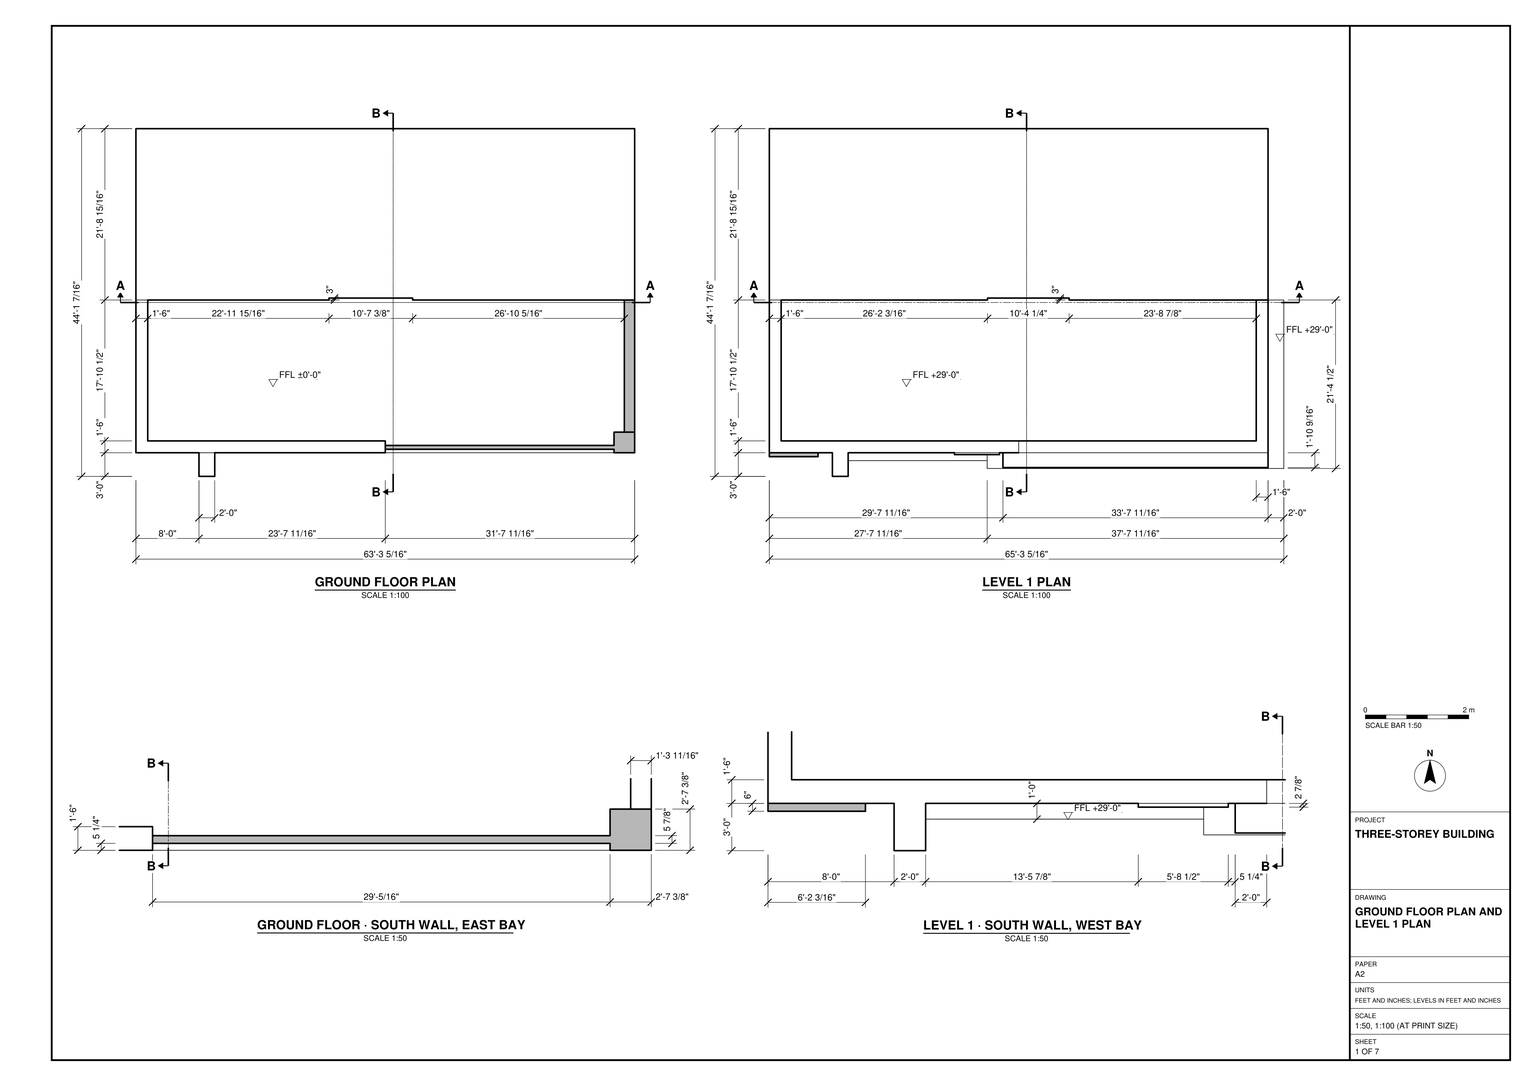
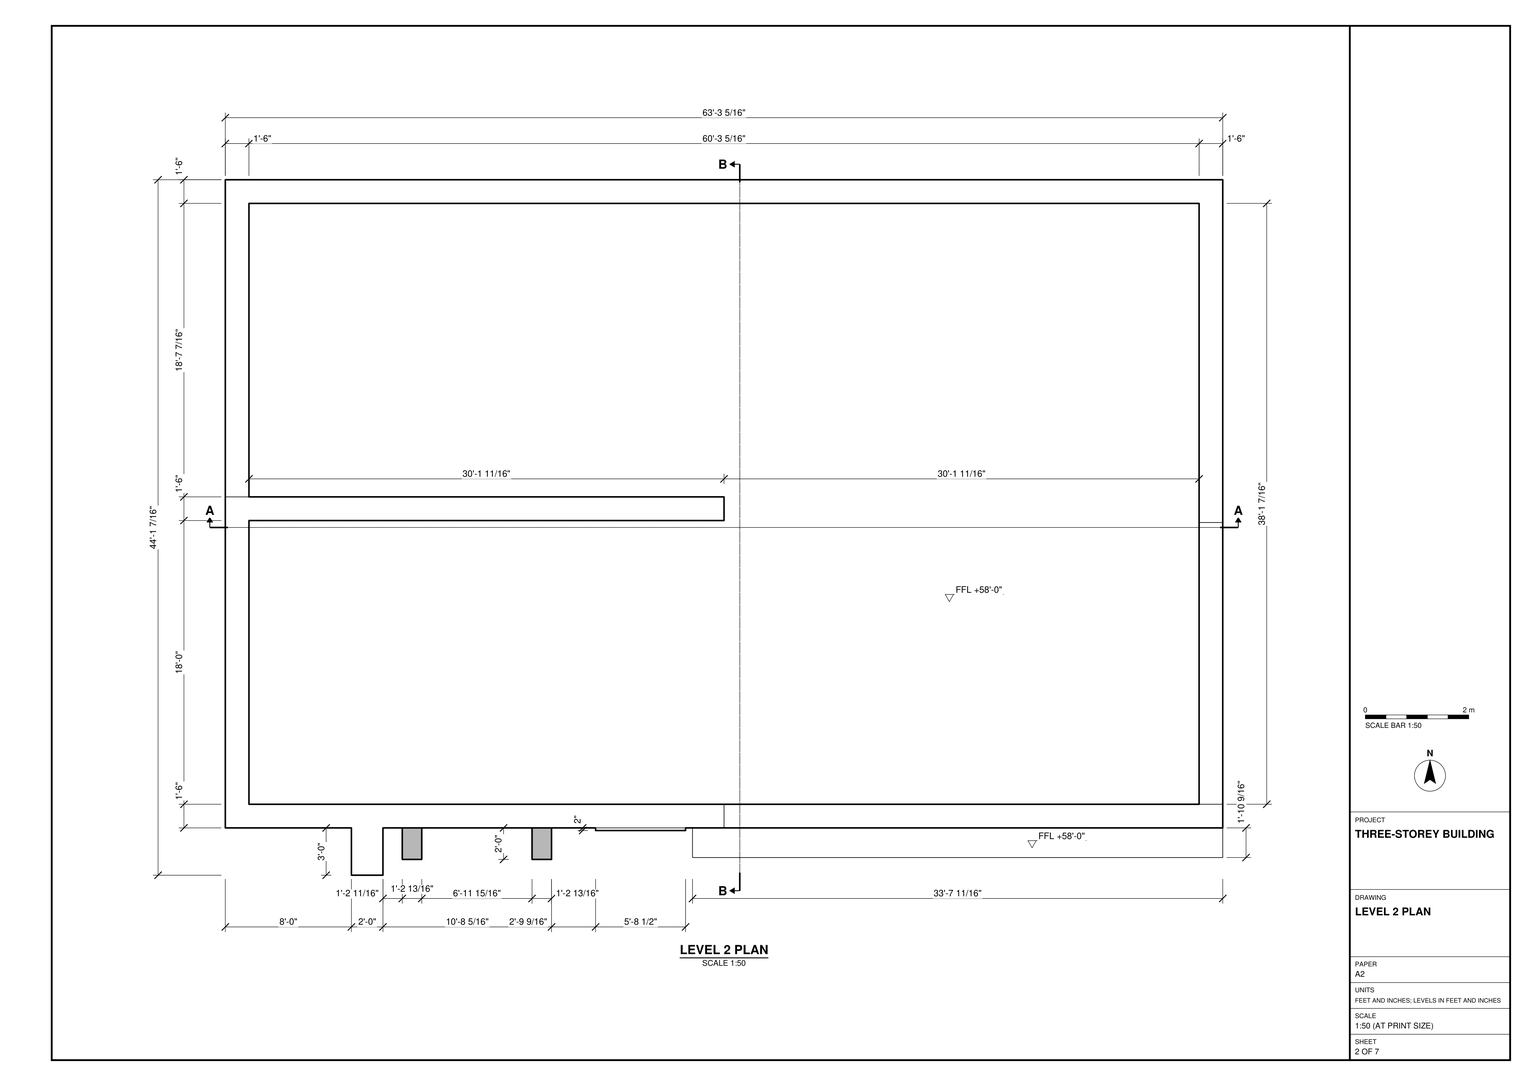
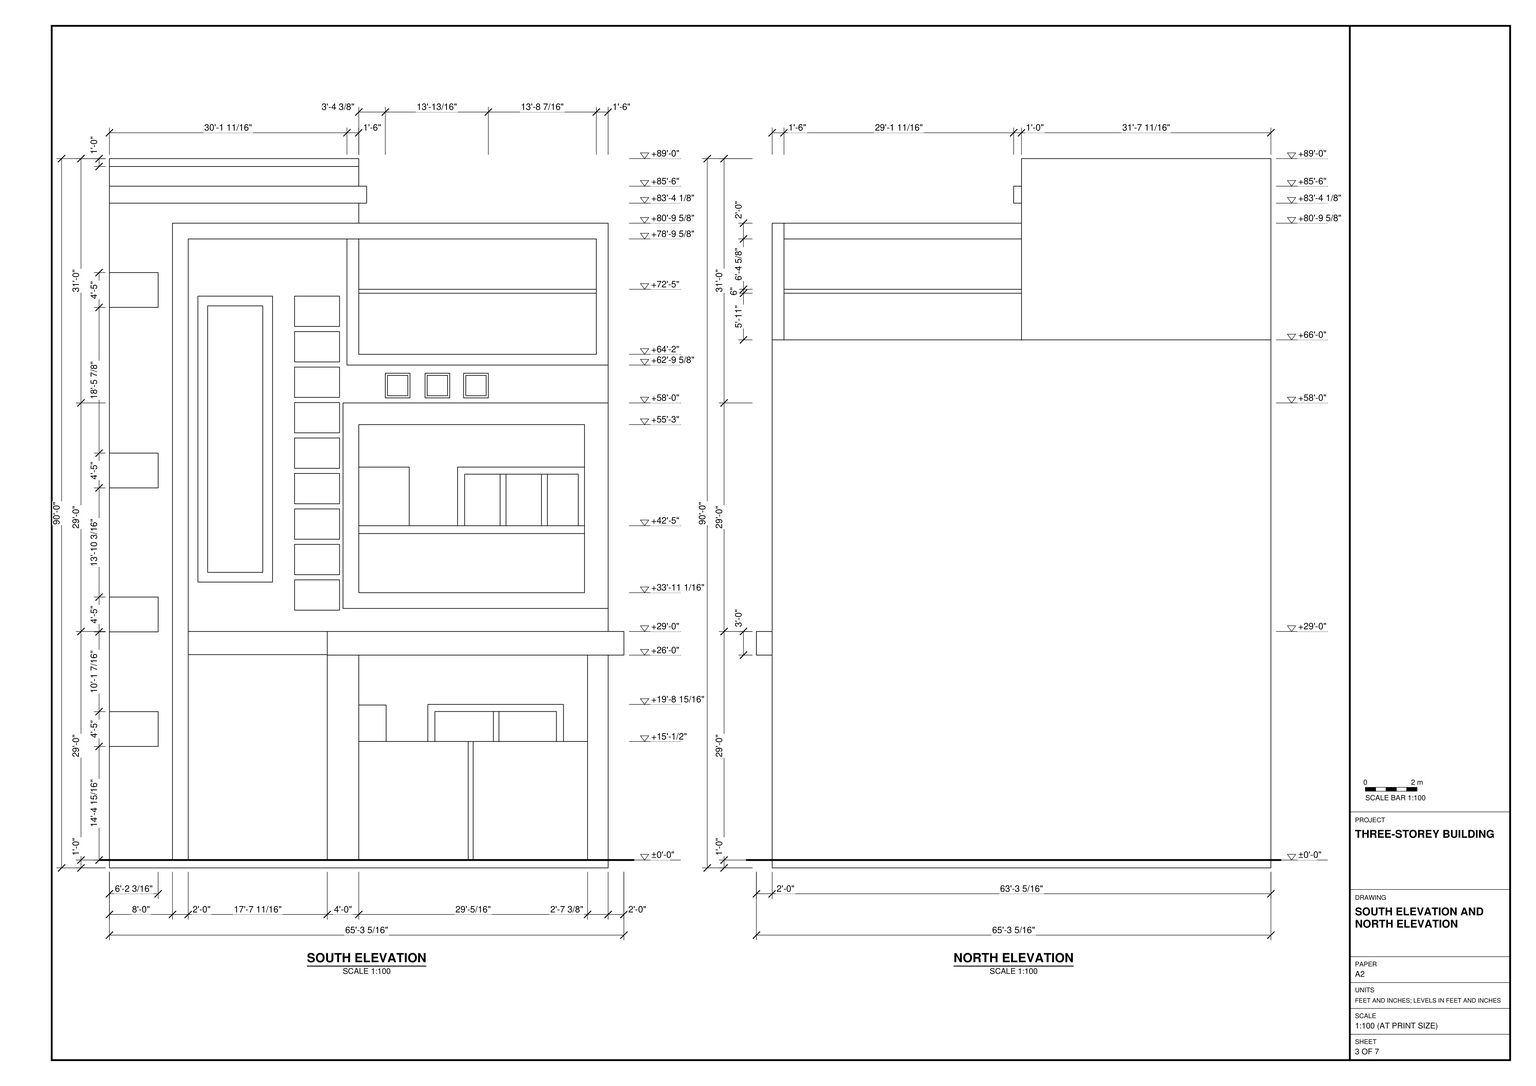
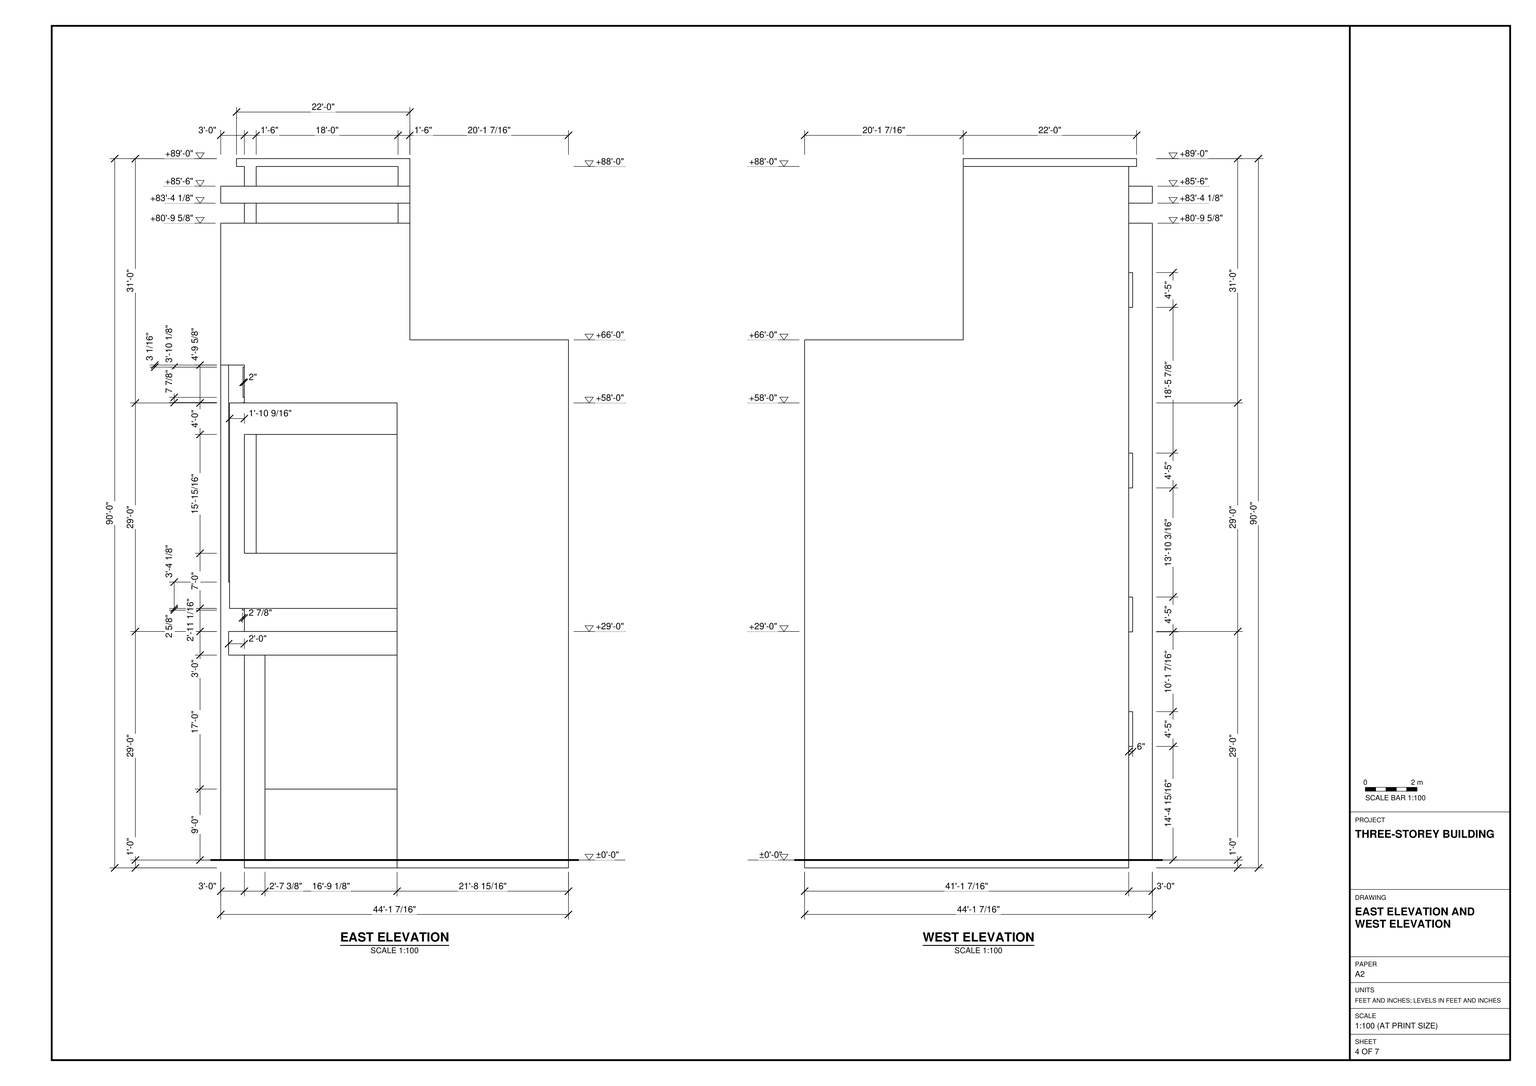
Build the three-storey building in SketchUp from task_files/diagram_01.pdf. Work in feet and inches. The overall extents, including projections, are 65'-3 5/16" east to west, 44'-1 7/16" north to south and 90'-0" from bottom to top. Set the finished floor levels at ±0'-0", +29'-0" and +58'-0".

Use the plans to lay out the slabs, walls and openings. Follow the wall thicknesses as drawn, including the 1'-6" perimeter walls on Level 2 and the thinner section of the ground-floor south wall at the east bay. On Level 2, run the interior wall from the west wall to the middle of the plan. Form the stepped roofline with the west portion higher than the east.

Use the south elevation and wall details to place the end pier, projecting floor band, window units and façade frames. Distinguish the tall narrow frame and vertical stack of panels on the west from the broad framed bays on the east. Include stairs, built-in joinery and main furniture only where shown. Decor and loose items may be any suitable library components.

Keep walls, slabs, roof elements and each furniture or joinery piece in separate groups or components, and use components for repeated parts. Save one SketchUp model as output_files/three_storey_building_with_stepped_roof_and_south_facade.skp.

# SketchUp Ruby script. Lengths in inches.
U = 1.inch
M = Sketchup.active_model
def pt(a) = Geom::Point3d.new(a.map { |v| v * U })
def face(e, loops, mat)
  f = e.add_face(loops[0].map { |a| pt(a) })
  loops[1..].each { |l| e.add_face(l.map { |a| pt(a) }).erase! }
  f.material = f.back_material = mat if mat
  f
end
# faces: each face lists its corners as indices into pts; further lists are holes
def faces(e, pts, list, mat = nil) = list.each { |f| face(e, (f[0].is_a?(Array) ? f : [f]).map { |l| l.map { |i| pts[i] } }, mat) }
# xy, xz, yz: faces in a plane at the given z, y or x. An outline is a flat list of corners, or four numbers for a rectangle; further outlines are holes
def ring(l) = l.size == 4 ? [[l[0], l[1]], [l[2], l[1]], [l[2], l[3]], [l[0], l[3]]] : l.each_slice(2).to_a
def flat(e, list, mat, &to3) = list.each { |f| face(e, (f[0].is_a?(Array) ? f : [f]).map { |l| ring(l).map { |u, v| to3.(u, v) } }, mat) }
def xy(e, z, list, mat = nil) = flat(e, list, mat) { |x, y| [x, y, z] }
def xz(e, y, list, mat = nil) = flat(e, list, mat) { |x, z| [x, y, z] }
def yz(e, x, list, mat = nil) = flat(e, list, mat) { |y, z| [x, y, z] }
def lines(e, pts, list) = list.each { |a, b| e.add_line(pt(pts[a]), pt(pts[b])) }
# prism: a flat outline (further loops are holes) pulled along v
def prism(e, loops, v, mat = nil)
  f = face(e, loops, mat); d = Geom::Vector3d.new(v.map { |x| x * U })
  f.pushpull(f.normal.samedirection?(d) ? d.length : -d.length)
end
def box(e, o, s, mat = nil) = prism(e, [[o, [o[0] + s[0], o[1], o[2]], [o[0] + s[0], o[1] + s[1], o[2]], [o[0], o[1] + s[1], o[2]]]], [0, 0, s[2]], mat)
def at(x, y, z, deg = 0) = Geom::Transformation.translation(pt([x, y, z])) * Geom::Transformation.rotation(ORIGIN, Z_AXIS, deg.degrees)
def axes(o, x, y, z) = Geom::Transformation.new([*x, 0, *y, 0, *z, 0, *pt(o).to_a, 1])
def part(name) = M.definitions.add(name)
# library, detail: a bought-in or finely detailed component or shape, given as its bounding box
def library(name, o, s) = part(name).tap { |d| box(d.entities, o, s) }
def detail(e, o, s) = box(e.add_group.entities, o, s)
def put(e, d, t, mat = nil) = e.add_instance(d, t).tap { |i| i.material = mat if mat }
def group(e, t, mat = nil) = e.add_group.tap { |g| g.transformation = t; g.material = mat if mat }.entities
root = M.entities
M.materials.add("[0006_Pink]").color = [153, 115, 121]
M.materials.add("[0007_MistyRose]").color = [209, 186, 184]
M.materials.add("[0012_Bisque]").color = [198, 177, 152]
M.materials.add("[0013_LightCoral]").color = [240, 128, 128]
M.materials.add("[0014_DarkSalmon]").color = [233, 150, 122]
M.materials.add("[0125_Plum]").color = [142, 103, 142]
M.materials.add("[0135_DarkGray]").color = [81, 81, 81]
M.materials.add("[0137_Black]").color = [0, 0, 0]
M.materials.add("[Cladding Siding Tan]").color = [162, 126, 95]
M.materials.add("[Metal Steel Textured White]").color = [191, 191, 191]
M.materials.add("[Stone Marble]").color = [143, 138, 136]
M.materials.add("[Translucent Glass Gray]").color = [128, 128, 128]
M.materials["[Translucent Glass Gray]"].alpha = 0.5
M.materials.add("[Translucent Glass Sky Reflection]").color = [126, 138, 183]
M.materials["[Translucent Glass Sky Reflection]"].alpha = 0.52
M.materials.add("[Wood Cherry Original]").color = [152, 86, 42]
M.materials.add("[Wood Veneer 01]").color = [120, 70, 37]
xy(root,0,[[0,36,759.3125,529.4375]],"[0006_Pink]")
xy(root,12,[[96,0,120,36],[0,36,0,268.5,18,268.5,18,54,379.656,54,379.656,36],[727.9375,36,759.3125,67.375],[379.656,41.253,727.9375,47.128],[743.625,67.375,759.3125,268.5],
  [0,268.5,0,529.4375,759.3125,529.4375,759.3125,268.5,421.298,268.5,421.298,271.5,293.923,271.5,293.923,268.5]],"[0006_Pink]")
xy(root,12,[[379.656,36,727.9375,41.253],[379.656,47.128,727.9375,47.128,727.9375,67.375,743.625,67.375,743.625,268.5,421.298,268.5,421.298,271.5,293.923,271.5,293.923,268.5,18,268.5,18,54,379.656,54]],"[Stone Marble]")
xy(root,120,[[743.625,67.375,759.3125,268.5]],"[0014_DarkSalmon]")
xy(root,184.965,[[0,30,74.1875,36]])
xy(root,192.5,[[379.656,41.253,727.9375,47.128]],"[0137_Black]")
xy(root,237.965,[[0,30,74.1875,36]])
xy(root,248,[[293.923,268.5,421.298,271.5]],"[Wood Cherry Original]")
xy(root,324,[[399.53,28.465,397.982,28.704,396.548,29.335,395.327,30.315,394.401,31.579,393.834,33.038,393.663,34.596,393.902,36.144,394.533,37.577,395.514,38.798,396.777,39.724,398.237,40.292,399.794,40.462,401.342,40.223,402.775,39.592,403.997,38.612,404.923,37.348,405.49,35.889,405.66,34.331,405.422,32.783,404.791,31.35,403.81,30.129,402.547,29.203,401.087,28.635],[495.53,28.465,493.982,28.704,492.548,29.335,491.327,30.315,490.401,31.579,489.834,33.038,489.663,34.596,489.902,36.144,490.533,37.577,491.514,38.798,492.777,39.724,494.237,40.292,495.794,40.462,497.342,40.223,498.775,39.592,499.997,38.612,500.923,37.348,501.49,35.889,501.66,34.331,501.422,32.783,500.791,31.35,499.81,30.129,498.547,29.203,497.087,28.635],[591.53,28.465,589.982,28.704,588.548,29.335,587.327,30.315,586.401,31.579,585.834,33.038,585.663,34.596,585.902,36.144,586.533,37.577,587.514,38.798,588.777,39.724,590.237,40.292,591.794,40.462,593.342,40.223,594.775,39.592,595.997,38.612,596.923,37.348,597.49,35.889,597.66,34.331,597.422,32.783,596.791,31.35,595.81,30.129,594.547,29.203,593.087,28.635],[687.53,28.465,685.982,28.704,684.548,29.335,683.327,30.315,682.401,31.579,681.834,33.038,681.663,34.596,681.902,36.144,682.533,37.577,683.514,38.798,684.777,39.724,686.237,40.292,687.794,40.462,689.342,40.223,690.775,39.592,691.997,38.612,692.923,37.348,693.49,35.889,693.66,34.331,693.422,32.783,692.791,31.35,691.81,30.129,690.547,29.203,689.087,28.635],[758.608,82.414,757.064,82.677,755.64,83.33,754.434,84.33,753.528,85.607,752.983,87.076,752.837,88.635,753.1,90.179,753.753,91.603,754.753,92.809,756.03,93.715,757.499,94.26,759.058,94.406,760.602,94.143,762.026,93.49,763.232,92.49,764.138,91.213,764.683,89.744,764.829,88.185,764.566,86.641,763.913,85.217,762.914,84.011,761.636,83.105,760.167,82.56],
  [758.608,158.539,757.064,158.802,755.64,159.455,754.434,160.455,753.528,161.732,752.983,163.201,752.837,164.76,753.1,166.304,753.753,167.728,754.753,168.934,756.03,169.84,757.499,170.385,759.058,170.531,760.602,170.268,762.026,169.615,763.232,168.615,764.138,167.338,764.683,165.869,764.829,164.31,764.566,162.766,763.913,161.342,762.914,160.136,761.636,159.23,760.167,158.685],[758.608,242.539,757.064,242.802,755.64,243.455,754.434,244.455,753.528,245.732,752.983,247.201,752.837,248.76,753.1,250.304,753.753,251.728,754.753,252.934,756.03,253.84,757.499,254.385,759.058,254.531,760.602,254.268,762.026,253.615,763.232,252.615,764.138,251.338,764.683,249.869,764.829,248.31,764.566,246.766,763.913,245.342,762.914,244.136,761.636,243.23,760.167,242.685]])
xy(root,324,[[[331.656,12,331.656,36,379.656,36,379.656,51.6875,727.9375,51.6875,727.9375,36,759.3125,36,759.3125,67.375,743.625,67.375,743.625,268.5,783.3125,268.5,783.3125,12],[591.53,28.465,593.087,28.635,594.547,29.203,595.81,30.129,596.791,31.35,597.422,32.783,597.66,34.331,597.49,35.889,596.923,37.348,595.997,38.612,594.775,39.592,593.342,40.223,591.794,40.462,590.237,40.292,588.777,39.724,587.514,38.798,586.533,37.577,585.902,36.144,585.663,34.596,585.834,33.038,586.401,31.579,587.327,30.315,588.548,29.335,589.982,28.704],[687.53,28.465,689.087,28.635,690.547,29.203,691.81,30.129,692.791,31.35,693.422,32.783,693.66,34.331,693.49,35.889,692.923,37.348,691.997,38.612,690.775,39.592,689.342,40.223,687.794,40.462,686.237,40.292,684.777,39.724,683.514,38.798,682.533,37.577,681.902,36.144,681.663,34.596,681.834,33.038,682.401,31.579,683.327,30.315,684.548,29.335,685.982,28.704],[399.53,28.465,401.087,28.635,402.547,29.203,403.81,30.129,404.791,31.35,405.422,32.783,405.66,34.331,405.49,35.889,404.923,37.348,403.997,38.612,402.775,39.592,401.342,40.223,399.794,40.462,398.237,40.292,396.777,39.724,395.514,38.798,394.533,37.577,393.902,36.144,393.663,34.596,393.834,33.038,394.401,31.579,395.327,30.315,396.548,29.335,397.982,28.704],[495.53,28.465,497.087,28.635,498.547,29.203,499.81,30.129,500.791,31.35,501.422,32.783,501.66,34.331,501.49,35.889,500.923,37.348,499.997,38.612,498.775,39.592,497.342,40.223,495.794,40.462,494.237,40.292,492.777,39.724,491.514,38.798,490.533,37.577,489.902,36.144,489.663,34.596,489.834,33.038,490.401,31.579,491.327,30.315,492.548,29.335,493.982,28.704],[758.608,242.539,760.167,242.685,761.636,243.23,762.914,244.136,763.913,245.342,764.566,246.766,764.829,248.31,764.683,249.869,764.138,251.338,763.232,252.615,762.026,253.615,760.602,254.268,759.058,254.531,757.499,254.385,756.03,253.84,754.753,252.934,753.753,251.728,753.1,250.304,752.837,248.76,752.983,247.201,753.528,245.732,754.434,244.455,755.64,243.455,757.064,242.802],[758.608,158.539,760.167,158.685,761.636,159.23,762.914,160.136,763.913,161.342,764.566,162.766,764.829,164.31,764.683,165.869,764.138,167.338,763.232,168.615,762.026,169.615,760.602,170.268,759.058,170.531,757.499,170.385,756.03,169.84,754.753,168.934,753.753,167.728,753.1,166.304,752.837,164.76,752.983,163.201,753.528,161.732,754.434,160.455,755.64,159.455,757.064,158.802],[758.608,82.414,760.167,82.56,761.636,83.105,762.914,84.011,763.913,85.217,764.566,86.641,764.829,88.185,764.683,89.744,764.138,91.213,763.232,92.49,762.026,93.49,760.602,94.143,759.058,94.406,757.499,94.26,756.03,93.715,754.753,92.809,753.753,91.603,753.1,90.179,752.837,88.635,752.983,87.076,753.528,85.607,754.434,84.33,755.64,83.33,757.064,82.677]]],"[Wood Veneer 01]")
xy(root,324.772,[[120,24,331.656,36]],"[0014_DarkSalmon]")
xy(root,348,[[379.656,51.6875,379.656,54,18,54,18,268.5,743.625,268.5,743.625,67.375,727.9375,67.375,727.9375,51.6875]],"[Wood Veneer 01]")
xy(root,359.402,[[0,30,74.1875,36]])
xy(root,360,[[379.656,36,379.656,54,741.3125,54,741.3125,268.5,759.3125,268.5,759.3125,36]])
xy(root,360,[[331.656,12,783.3125,12,783.3125,268.5,759.3125,268.5,759.3125,36,331.656,36],[120,24,331.656,36]],"[0014_DarkSalmon]")
xy(root,360,[[18,54,741.3125,54,741.3125,268.5,456.436,268.5,456.436,271.5,332.186,271.5,332.186,268.5,18,268.5]],"[Stone Marble]")
xy(root,392.443,[[281.876,33.125,350.376,36]],"[0014_DarkSalmon]")
xy(root,395.0625,[[355.656,13.4375,759.3125,36]],"[0014_DarkSalmon]")
xy(root,412.402,[[0,30,74.1875,36]])
xy(root,419.0625,[[379.656,13.4375,723.3125,24.419],[379.656,24.419,723.3125,24.719],[379.656,24.719,723.3125,24.739]])
xy(root,419.0625,[[379.656,24.739,723.3125,24.739,723.3125,36,741.3125,36,741.3125,54,379.656,54]],"[0014_DarkSalmon]")
xy(root,435.193,[[134.717,12,248.342,36]],"[0135_DarkGray]")
xy(root,438.568,[[281.876,33.125,350.376,36]],"[0014_DarkSalmon]")
xy(root,446.443,[[281.876,33.125,350.376,36]],"[0014_DarkSalmon]")
xy(root,450.031,[[149.555,12,233.504,36]],"[0135_DarkGray]")
xy(root,479.0625,[[741.3125,36,759.3125,268.5]],"[0014_DarkSalmon]")
xy(root,492.568,[[281.876,33.125,350.376,36]],"[0014_DarkSalmon]")
xy(root,500.443,[[281.876,34,350.376,36]])
xy(root,515.0625,[[379.656,24.419,723.3125,24.719],[379.656,24.719,723.3125,24.739]])
xy(root,546.568,[[281.876,34,350.376,36]],"[0014_DarkSalmon]")
xy(root,554.443,[[281.876,34,350.376,36]])
xy(root,578.59,[[0,30,74.1875,36]])
xy(root,600.568,[[281.876,34,350.376,36]],"[0014_DarkSalmon]")
xy(root,608.443,[[281.876,34,350.376,36]],"[0014_DarkSalmon]")
xy(root,610.25,[[332.186,268.5,456.436,271.5]],"[Wood Cherry Original]")
xy(root,631.59,[[0,30,74.1875,36]])
xy(root,654.568,[[281.876,34,350.376,36]],"[0014_DarkSalmon]")
xy(root,660,[[723.3125,36,759.3125,268.5]],"[Wood Veneer 01]")
xy(root,662.443,[[281.876,34,350.376,36]],"[0014_DarkSalmon]")
xy(root,675,[[435.209,17.737,433.65,17.881,432.181,18.425,430.902,19.329,429.901,20.534,429.247,21.957,428.983,23.501,429.127,25.061,429.67,26.53,430.575,27.808,431.78,28.809,433.203,29.464,434.747,29.728,436.307,29.583,437.776,29.04,439.054,28.135,440.055,26.93,440.71,25.507,440.974,23.963,440.829,22.404,440.286,20.935,439.381,19.656,438.176,18.656,436.753,18.001],[483.209,17.737,481.65,17.881,480.181,18.425,478.902,19.329,477.901,20.534,477.247,21.957,476.983,23.501,477.127,25.061,477.67,26.53,478.575,27.808,479.78,28.809,481.203,29.464,482.747,29.728,484.307,29.583,485.776,29.04,487.054,28.135,488.055,26.93,488.71,25.507,488.974,23.963,488.829,22.404,488.286,20.935,487.381,19.656,486.176,18.656,484.753,18.001],[531.209,17.737,529.65,17.881,528.181,18.425,526.902,19.329,525.901,20.534,525.247,21.957,524.983,23.501,525.127,25.061,525.67,26.53,526.575,27.808,527.78,28.809,529.203,29.464,530.747,29.728,532.307,29.583,533.776,29.04,535.054,28.135,536.055,26.93,536.71,25.507,536.974,23.963,536.829,22.404,536.286,20.935,535.381,19.656,534.176,18.656,532.753,18.001],[579.209,17.737,577.65,17.881,576.181,18.425,574.902,19.329,573.901,20.534,573.247,21.957,572.983,23.501,573.127,25.061,573.67,26.53,574.575,27.808,575.78,28.809,577.203,29.464,578.747,29.728,580.307,29.583,581.776,29.04,583.054,28.135,584.055,26.93,584.71,25.507,584.974,23.963,584.829,22.404,584.286,20.935,583.381,19.656,582.176,18.656,580.753,18.001],[627.209,17.737,625.65,17.881,624.181,18.425,622.902,19.329,621.901,20.534,621.247,21.957,620.983,23.501,621.127,25.061,621.67,26.53,622.575,27.808,623.78,28.809,625.203,29.464,626.747,29.728,628.307,29.583,629.776,29.04,631.054,28.135,632.055,26.93,632.71,25.507,632.974,23.963,632.829,22.404,632.286,20.935,631.381,19.656,630.176,18.656,628.753,18.001],
  [675.209,17.737,673.65,17.881,672.181,18.425,670.902,19.329,669.901,20.534,669.247,21.957,668.983,23.501,669.127,25.061,669.67,26.53,670.575,27.808,671.78,28.809,673.203,29.464,674.747,29.728,676.307,29.583,677.776,29.04,679.054,28.135,680.055,26.93,680.71,25.507,680.974,23.963,680.829,22.404,680.286,20.935,679.381,19.656,678.176,18.656,676.753,18.001],[723.3125,17.754,723.3125,29.676,724.307,29.583,725.776,29.04,727.054,28.135,728.055,26.93,728.71,25.507,728.974,23.963,728.829,22.404,728.286,20.935,727.381,19.656,726.176,18.656,724.753,18.001]])
xy(root,675,[[[379.656,13.4375,723.3125,36],[675.209,17.737,676.753,18.001,678.176,18.656,679.381,19.656,680.286,20.935,680.829,22.404,680.974,23.963,680.71,25.507,680.055,26.93,679.054,28.135,677.776,29.04,676.307,29.583,674.747,29.728,673.203,29.464,671.78,28.809,670.575,27.808,669.67,26.53,669.127,25.061,668.983,23.501,669.247,21.957,669.901,20.534,670.902,19.329,672.181,18.425,673.65,17.881],[627.209,17.737,628.753,18.001,630.176,18.656,631.381,19.656,632.286,20.935,632.829,22.404,632.974,23.963,632.71,25.507,632.055,26.93,631.054,28.135,629.776,29.04,628.307,29.583,626.747,29.728,625.203,29.464,623.78,28.809,622.575,27.808,621.67,26.53,621.127,25.061,620.983,23.501,621.247,21.957,621.901,20.534,622.902,19.329,624.181,18.425,625.65,17.881],[579.209,17.737,580.753,18.001,582.176,18.656,583.381,19.656,584.286,20.935,584.829,22.404,584.974,23.963,584.71,25.507,584.055,26.93,583.054,28.135,581.776,29.04,580.307,29.583,578.747,29.728,577.203,29.464,575.78,28.809,574.575,27.808,573.67,26.53,573.127,25.061,572.983,23.501,573.247,21.957,573.901,20.534,574.902,19.329,576.181,18.425,577.65,17.881],[435.209,17.737,436.753,18.001,438.176,18.656,439.381,19.656,440.286,20.935,440.829,22.404,440.974,23.963,440.71,25.507,440.055,26.93,439.054,28.135,437.776,29.04,436.307,29.583,434.747,29.728,433.203,29.464,431.78,28.809,430.575,27.808,429.67,26.53,429.127,25.061,428.983,23.501,429.247,21.957,429.901,20.534,430.902,19.329,432.181,18.425,433.65,17.881],[531.209,17.737,532.753,18.001,534.176,18.656,535.381,19.656,536.286,20.935,536.829,22.404,536.974,23.963,536.71,25.507,536.055,26.93,535.054,28.135,533.776,29.04,532.307,29.583,530.747,29.728,529.203,29.464,527.78,28.809,526.575,27.808,525.67,26.53,525.127,25.061,524.983,23.501,525.247,21.957,525.901,20.534,526.902,19.329,528.181,18.425,529.65,17.881],[483.209,17.737,484.753,18.001,486.176,18.656,487.381,19.656,488.286,20.935,488.829,22.404,488.974,23.963,488.71,25.507,488.055,26.93,487.054,28.135,485.776,29.04,484.307,29.583,482.747,29.728,481.203,29.464,479.78,28.809,478.575,27.808,477.67,26.53,477.127,25.061,476.983,23.501,477.247,21.957,477.901,20.534,478.902,19.329,480.181,18.425,481.65,17.881]]],"[Wood Veneer 01]")
xy(root,694,[[379.656,36,379.656,54,18,54,18,268.5,723.3125,268.5,723.3125,36]],"[Wood Veneer 01]")
xy(root,708,[[379.656,36,759.3125,54],[18,54,741.3125,54,741.3125,511.4375,18,511.4375,18,288,379.656,288,379.656,270,18,270]])
xy(root,708,[[355.656,13.4375,759.3125,36]],"[0014_DarkSalmon]")
xy(root,708.568,[[281.876,34,350.376,36]],"[0014_DarkSalmon]")
xy(root,716.443,[[281.876,34,350.376,36]],"[0014_DarkSalmon]")
xy(root,762.568,[[281.876,34,350.376,36]],"[0014_DarkSalmon]")
xy(root,765.648,[[361.656,0,759.3125,36]],"[0014_DarkSalmon]")
xy(root,770.443,[[281.876,34,350.376,36]],"[0014_DarkSalmon]")
xy(root,782,[[379.656,17.68,741.3125,18],[379.656,18,741.3125,54]])
xy(root,782,[[379.656,0,741.3125,17.68]],"[0014_DarkSalmon]")
xy(root,804,[[0,288,18,288,18,511.4375,741.3125,511.4375,741.3125,288,759.3125,288,759.3125,529.4375,0,529.4375]],"[0007_MistyRose]")
xy(root,816.568,[[281.876,34,350.376,36]])
xy(root,824.443,[[281.876,34,350.376,36]],"[0014_DarkSalmon]")
xy(root,853.465,[[0,30,74.1875,36]])
xy(root,855.729,[[149.555,12,233.504,36]],"[0135_DarkGray]")
xy(root,870.568,[[281.876,34,350.376,36]])
xy(root,870.568,[[134.717,12,248.342,36]],"[0135_DarkGray]")
xy(root,875,[[379.656,17.68,741.3125,18]])
xy(root,906.465,[[0,30,74.1875,36]])
xy(root,957.648,[[361.656,0,379.656,36],[161.674,14.482,160.143,14.812,158.749,15.526,157.588,16.578,156.739,17.893,156.259,19.384,156.181,20.949,156.51,22.48,157.225,23.874,158.276,25.035,159.592,25.884,161.083,26.364,162.648,26.442,164.179,26.113,165.573,25.398,166.734,24.347,167.583,23.031,168.063,21.54,168.141,19.975,167.811,18.444,167.097,17.05,166.045,15.889,164.73,15.04,163.239,14.56],[244.487,14.482,242.956,14.812,241.562,15.526,240.401,16.578,239.551,17.893,239.071,19.384,238.993,20.949,239.323,22.48,240.038,23.874,241.089,25.035,242.405,25.884,243.896,26.364,245.46,26.442,246.991,26.113,248.385,25.398,249.546,24.347,250.396,23.031,250.876,21.54,250.954,19.975,250.624,18.444,249.909,17.05,248.858,15.889,247.542,15.04,246.051,14.56],[336.549,14.482,335.018,14.812,333.624,15.526,332.463,16.578,331.614,17.893,331.134,19.384,331.056,20.949,331.385,22.48,332.1,23.874,333.151,25.035,334.467,25.884,335.958,26.364,337.523,26.442,339.054,26.113,340.448,25.398,341.609,24.347,342.458,23.031,342.938,21.54,343.016,19.975,342.686,18.444,341.972,17.05,340.92,15.889,339.605,15.04,338.114,14.56],[422.987,14.482,421.456,14.812,420.062,15.526,418.901,16.578,418.051,17.893,417.571,19.384,417.493,20.949,417.823,22.48,418.538,23.874,419.589,25.035,420.905,25.884,422.396,26.364,423.96,26.442,425.491,26.113,426.885,25.398,428.046,24.347,428.896,23.031,429.376,21.54,429.454,19.975,429.124,18.444,428.409,17.05,427.358,15.889,426.042,15.04,424.551,14.56],
  [564.299,14.482,562.768,14.812,561.374,15.526,560.213,16.578,559.364,17.893,558.884,19.384,558.806,20.949,559.135,22.48,559.85,23.874,560.901,25.035,562.217,25.884,563.708,26.364,565.273,26.442,566.804,26.113,568.198,25.398,569.359,24.347,570.208,23.031,570.688,21.54,570.766,19.975,570.436,18.444,569.722,17.05,568.67,15.889,567.355,15.04,565.864,14.56],[702.674,14.482,701.143,14.812,699.749,15.526,698.588,16.578,697.739,17.893,697.259,19.384,697.181,20.949,697.51,22.48,698.225,23.874,699.276,25.035,700.592,25.884,702.083,26.364,703.648,26.442,705.179,26.113,706.573,25.398,707.734,24.347,708.583,23.031,709.063,21.54,709.141,19.975,708.811,18.444,708.097,17.05,707.045,15.889,705.73,15.04,704.239,14.56]])
xy(root,957.648,[[[120,0,361.656,36],[336.549,14.482,338.114,14.56,339.605,15.04,340.92,15.889,341.972,17.05,342.686,18.444,343.016,19.975,342.938,21.54,342.458,23.031,341.609,24.347,340.448,25.398,339.054,26.113,337.523,26.442,335.958,26.364,334.467,25.884,333.151,25.035,332.1,23.874,331.385,22.48,331.056,20.949,331.134,19.384,331.614,17.893,332.463,16.578,333.624,15.526,335.018,14.812],[161.674,14.482,163.239,14.56,164.73,15.04,166.045,15.889,167.097,17.05,167.811,18.444,168.141,19.975,168.063,21.54,167.583,23.031,166.734,24.347,165.573,25.398,164.179,26.113,162.648,26.442,161.083,26.364,159.592,25.884,158.276,25.035,157.225,23.874,156.51,22.48,156.181,20.949,156.259,19.384,156.739,17.893,157.588,16.578,158.749,15.526,160.143,14.812],[244.487,14.482,246.051,14.56,247.542,15.04,248.858,15.889,249.909,17.05,250.624,18.444,250.954,19.975,250.876,21.54,250.396,23.031,249.546,24.347,248.385,25.398,246.991,26.113,245.46,26.442,243.896,26.364,242.405,25.884,241.089,25.035,240.038,23.874,239.323,22.48,238.993,20.949,239.071,19.384,239.551,17.893,240.401,16.578,241.562,15.526,242.956,14.812]],[[379.656,0,741.3125,36],[422.987,14.482,424.551,14.56,426.042,15.04,427.358,15.889,428.409,17.05,429.124,18.444,429.454,19.975,429.376,21.54,428.896,23.031,428.046,24.347,426.885,25.398,425.491,26.113,423.96,26.442,422.396,26.364,420.905,25.884,419.589,25.035,418.538,23.874,417.823,22.48,417.493,20.949,417.571,19.384,418.051,17.893,418.901,16.578,420.062,15.526,421.456,14.812],[564.299,14.482,565.864,14.56,567.355,15.04,568.67,15.889,569.722,17.05,570.436,18.444,570.766,19.975,570.688,21.54,570.208,23.031,569.359,24.347,568.198,25.398,566.804,26.113,565.273,26.442,563.708,26.364,562.217,25.884,560.901,25.035,559.85,23.874,559.135,22.48,558.806,20.949,558.884,19.384,559.364,17.893,560.213,16.578,561.374,15.526,562.768,14.812],[702.674,14.482,704.239,14.56,705.73,15.04,707.045,15.889,708.097,17.05,708.811,18.444,709.141,19.975,709.063,21.54,708.583,23.031,707.734,24.347,706.573,25.398,705.179,26.113,703.648,26.442,702.083,26.364,700.592,25.884,699.276,25.035,698.225,23.874,697.51,22.48,697.181,20.949,697.259,19.384,697.739,17.893,698.588,16.578,699.749,15.526,701.143,14.812]],[379.656,270,741.3125,288]],"[0014_DarkSalmon]")
xy(root,962.165,[[389.456,36,410.269,270],[443.456,36,464.269,270],[497.456,36,518.269,270],[551.456,36,572.269,270],[605.456,36,626.269,270],
  [659.456,36,680.269,270],[713.456,36,734.269,270]],"[0014_DarkSalmon]")
xy(root,977.603,[[389.456,36,410.269,270],[443.456,36,464.269,270],[497.456,36,518.269,270],[551.456,36,572.269,270],[605.456,36,626.269,270],
  [659.456,36,680.269,270],[713.456,36,734.269,270]],"[0014_DarkSalmon]")
xy(root,981.648,[[96,0,759.3125,0,759.3125,288,379.656,288,379.656,270,741.3125,270,741.3125,36,96,36]],"[0014_DarkSalmon]")
xy(root,1012.128,[[0,0,0,36,379.656,36,379.656,288,391.656,288,391.656,0]],"[0013_LightCoral]")
xy(root,1037.995,[[0,0,391.656,0,391.656,288,379.656,288,379.656,36,0,36]],"[0013_LightCoral]")
xy(root,1068,[[18,54,379.656,270]])
xy(root,1068,[[0,24,379.656,36]],"[0013_LightCoral]")
xy(root,1080,[[0,24,379.656,288]],"[0013_LightCoral]")
xz(root,0,[[0,1012.128,391.656,1037.995]],"[0013_LightCoral]")
xz(root,0,[[96,12,120,12,120,957.648,741.3125,957.648,741.3125,782,379.656,782,379.656,957.648,361.656,957.648,361.656,765.648,759.3125,765.648,759.3125,981.648,96,981.648]],"[0014_DarkSalmon]")
xz(root,12,[[331.656,324,783.3125,360]],"[0014_DarkSalmon]")
xz(root,12,[[[134.717,435.193,248.342,870.568],[149.555,450.031,233.504,855.729]]],"[0135_DarkGray]")
xz(root,13.4375,[[[355.656,395.0625,759.3125,708],[379.656,419.0625,723.3125,675]]],"[0014_DarkSalmon]")
xz(root,17.68,[[379.656,782,741.3125,875]],"[Translucent Glass Gray]")
xz(root,18,[[379.656,782,741.3125,875]],"[Translucent Glass Gray]")
xz(root,24,[[0,1068,379.656,1080]],"[0013_LightCoral]")
xz(root,24,[[120,324.772,331.656,360]],"[0014_DarkSalmon]")
xz(root,24.419,[[379.656,419.0625,723.3125,515.0625]],"[Translucent Glass Gray]")
xz(root,24.719,[[379.656,419.0625,723.3125,515.0625]])
xz(root,24.739,[[379.656,419.0625,723.3125,515.0625]],"[Translucent Glass Gray]")
xz(root,30,[[0,184.965,74.1875,237.965],[0,359.402,74.1875,412.402],[0,578.59,74.1875,631.59],[0,853.465,74.1875,906.465]])
xz(root,33.125,[[281.876,392.443,350.376,438.568],[281.876,446.443,350.376,492.568]],"[0014_DarkSalmon]")
xz(root,34,[[281.876,500.443,350.376,546.568],[281.876,554.443,350.376,600.568],[281.876,608.443,350.376,654.568],[281.876,662.443,350.376,708.568],[281.876,716.443,350.376,762.568],
  [281.876,770.443,350.376,816.568],[281.876,824.443,350.376,870.568]],"[0014_DarkSalmon]")
xz(root,36,[[0,184.965,74.1875,237.965],[120,324.772,331.656,360],[0,359.402,74.1875,412.402],[355.656,395.0625,379.656,419.0625],[[134.717,435.193,248.342,870.568],[149.555,450.031,233.504,855.729]],
  [0,578.59,74.1875,631.59],[[420.05,715.649,457.612,753.212],[423.328,718.927,454.334,749.934]],[[480.55,715.649,518.112,753.212],[483.828,718.927,514.834,749.934]],[[539.3,715.649,576.862,753.212],[542.578,718.927,573.584,749.934]],[423.328,718.927,454.334,749.934],
  [483.828,718.927,514.834,749.934],[542.578,718.927,573.584,749.934],[0,853.465,74.1875,906.465],[0,1012.128,379.656,1037.995]])
xz(root,36,[[0,12,96,12,96,981.648,379.656,981.648,379.656,1012.128,0,1012.128,0,906.465,74.1875,906.465,74.1875,853.465,0,853.465,0,631.59,74.1875,631.59,74.1875,578.59,0,578.59,0,412.402,74.1875,412.402,74.1875,359.402,0,359.402,0,237.965,74.1875,237.965,74.1875,184.965,0,184.965],[120,12,331.656,324.772]],"[0012_Bisque]")
xz(root,36,[[[120,360,759.3125,360,759.3125,395.0625,355.656,395.0625,355.656,708,759.3125,708,759.3125,765.648,361.656,765.648,361.656,957.648,120,957.648],[134.717,435.193,248.342,870.568],[281.876,824.443,350.376,870.568],[281.876,770.443,350.376,816.568],[281.876,716.443,350.376,762.568],[281.876,662.443,350.376,708.568],[281.876,608.443,350.376,654.568],[281.876,554.443,350.376,600.568],[281.876,500.443,350.376,546.568],[281.876,446.443,350.376,492.568],[281.876,392.443,350.376,438.568],[539.3,715.649,576.862,753.212],[420.05,715.649,457.612,753.212],[480.55,715.649,518.112,753.212]],[0,1037.995,379.656,1068]],"[0013_LightCoral]")
xz(root,36,[[723.3125,419.0625,723.3125,660,759.3125,660,759.3125,479.0625,741.3125,479.0625,741.3125,419.0625],[[379.656,957.648,741.3125,981.648],[389.456,962.165,410.269,977.603],[443.456,962.165,464.269,977.603],[497.456,962.165,518.269,977.603],[551.456,962.165,572.269,977.603],[605.456,962.165,626.269,977.603],[659.456,962.165,680.269,977.603],[713.456,962.165,734.269,977.603]]],"[0014_DarkSalmon]")
xz(root,36,[[379.656,675,723.3125,694]],"[0125_Plum]")
xz(root,36,[[331.656,12,379.656,324],[727.9375,12,759.3125,324]],"[0135_DarkGray]")
xz(root,36,[[0,0,759.3125,12]],"[Stone Marble]")
xz(root,36,[[149.555,450.031,233.504,855.729]],"[Translucent Glass Gray]")
xz(root,41.253,[[546.257,12,553.797,192.5]],"[0137_Black]")
xz(root,41.253,[[379.656,12,546.257,192.5],[553.797,12,727.9375,192.5]],"[Cladding Siding Tan]")
xz(root,47.128,[[379.656,12,727.9375,192.5]],"[Cladding Siding Tan]")
xz(root,51.6875,[[379.656,324,727.9375,348]],"[0125_Plum]")
xz(root,54,[[18,708,18,1068,379.656,1068,379.656,782,741.3125,782,741.3125,708]])
xz(root,54,[[379.656,360,741.3125,419.0625]],"[0014_DarkSalmon]")
xz(root,54,[[18,12,379.656,348],[18,360,379.656,694]],"[0125_Plum]")
xz(root,67.375,[[743.625,12,759.3125,120]],"[0006_Pink]")
xz(root,67.375,[[727.9375,12,727.9375,348,743.625,348,743.625,324,759.3125,324,759.3125,120,743.625,120,743.625,12]],"[0135_DarkGray]")
xz(root,268.5,[[743.625,324,759.3125,348],[759.3125,324,783.3125,360],[741.3125,360,759.3125,479.0625],[723.3125,660,759.3125,696],[18,694,723.3125,696]])
xz(root,268.5,[[743.625,12,759.3125,120]],"[0006_Pink]")
xz(root,268.5,[[[18,12,293.923,12,293.923,248,421.298,248,421.298,12,743.625,12,743.625,120,759.3125,120,759.3125,324,743.625,324,743.625,348,18,348],[484.775,113.621,691.338,248.933]],[[18,360,332.186,360,332.186,610.25,456.436,610.25,456.436,360,741.3125,360,741.3125,479.0625,759.3125,479.0625,759.3125,660,723.3125,660,723.3125,694,18,694],[530.076,479,724.576,610.25]]],"[0125_Plum]")
xz(root,268.5,[[[484.775,113.621,691.338,248.933],[495.549,124.394,680.564,238.16]],[584.633,124.394,593.05,238.16],[[530.076,479,724.576,610.25],[540.81,489.733,713.843,599.517]],[594.81,489.733,603.81,599.517],[657.81,489.733,666.81,599.517]],"[0137_Black]")
xz(root,268.5,[[495.549,124.394,584.633,238.16],[593.05,124.394,680.564,238.16],[540.81,489.733,594.81,599.517],[603.81,489.733,657.81,599.517],[666.81,489.733,713.843,599.517]],"[Translucent Glass Sky Reflection]")
xz(root,270,[[389.456,962.165,410.269,977.603]])
xz(root,270,[[18,708,379.656,1068]],"[0013_LightCoral]")
xz(root,270,[[[379.656,957.648,741.3125,981.648],[389.456,962.165,410.269,977.603],[443.456,962.165,464.269,977.603],[497.456,962.165,518.269,977.603],[551.456,962.165,572.269,977.603],[605.456,962.165,626.269,977.603],[659.456,962.165,680.269,977.603],[713.456,962.165,734.269,977.603]]],"[0014_DarkSalmon]")
xz(root,271.5,[[293.923,12,421.298,248],[332.186,360,456.436,610.25]],"[Wood Cherry Original]")
xz(root,288,[[18,708,18,804,0,804,0,1080,379.656,1080,379.656,708],[379.656,1012.128,391.656,1037.995]],"[0013_LightCoral]")
xz(root,288,[[741.3125,804,759.3125,981.648],[379.656,957.648,741.3125,981.648]],"[0014_DarkSalmon]")
xz(root,511.4375,[[18,708,741.3125,804]],"[0007_MistyRose]")
xz(root,529.4375,[[0,0,759.3125,12]],"[0006_Pink]")
xz(root,529.4375,[[0,12,759.3125,804]],"[0007_MistyRose]")
yz(root,0,[[30,184.965,36,237.965],[30,359.402,36,412.402],[30,578.59,36,631.59],[30,853.465,36,906.465]])
yz(root,0,[[36,0,529.4375,12]],"[0006_Pink]")
yz(root,0,[[36,12,36,1068,288,1068,288,804,529.4375,804,529.4375,12]],"[0007_MistyRose]")
yz(root,0,[[0,1012.128,36,1037.995],[24,1068,288,1080]],"[0013_LightCoral]")
yz(root,18,[[54,708,270,1068]])
yz(root,18,[[288,708,511.4375,804]],"[0007_MistyRose]")
yz(root,18,[[54,12,268.5,348],[54,360,268.5,694]],"[0125_Plum]")
yz(root,74.1875,[[30,184.965,36,237.965],[30,359.402,36,412.402],[30,578.59,36,631.59],[30,853.465,36,906.465]])
yz(root,96,[[0,12,36,981.648]],"[0014_DarkSalmon]")
yz(root,120,[[24,324.772,36,360]])
yz(root,120,[[0,12,36,12,36,324.772,24,324.772,24,360,36,360,36,957.648,0,957.648]],"[0014_DarkSalmon]")
yz(root,134.717,[[12,435.193,36,870.568]],"[0135_DarkGray]")
yz(root,149.555,[[12,450.031,36,855.729]],"[0135_DarkGray]")
yz(root,233.504,[[12,450.031,36,855.729]],"[0135_DarkGray]")
yz(root,248.342,[[12,435.193,36,870.568]],"[0135_DarkGray]")
yz(root,281.876,[[33.125,392.443,36,438.568],[33.125,446.443,36,492.568],[34,500.443,36,546.568],[34,554.443,36,600.568],[34,608.443,36,654.568],
  [34,662.443,36,708.568],[34,716.443,36,762.568],[34,770.443,36,816.568],[34,824.443,36,870.568]],"[0014_DarkSalmon]")
yz(root,293.923,[[268.5,12,271.5,248]],"[Wood Cherry Original]")
yz(root,331.656,[[12,324,12,360,24,360,24,324.772,36,324.772,36,324],[24,324.772,36,360]])
yz(root,332.186,[[268.5,360,271.5,610.25]],"[Wood Cherry Original]")
yz(root,350.376,[[34,770.443,36,816.568],[34,824.443,36,870.568]])
yz(root,350.376,[[33.125,392.443,36,438.568],[33.125,446.443,36,492.568],[34,500.443,36,546.568],[34,554.443,36,600.568],[34,608.443,36,654.568],
  [34,662.443,36,708.568],[34,716.443,36,762.568]],"[0014_DarkSalmon]")
yz(root,355.656,[[13.4375,395.0625,36,708]],"[0014_DarkSalmon]")
yz(root,361.656,[[0,765.648,36,957.648]],"[0014_DarkSalmon]")
yz(root,379.656,[[24.419,419.0625,24.719,419.0625,24.719,509.114,24.419,509.111],[24.719,419.0625,24.739,509.114],[24.419,509.111,24.419,509.114,24.719,509.114],[24.419,509.114,24.719,515.0625],[24.719,509.114,24.739,515.0625],
  [17.68,782,18,875],[18,875,17.224,875.102,16.5,875.402,15.879,875.879,15.402,876.5,15.102,877.224,15,878,15.102,878.776,15.402,879.5,15.879,880.121,16.5,880.598,17.224,880.898,18,881,18.776,880.898,19.5,880.598,20.121,880.121,20.598,879.5,20.898,878.776,21,878,20.898,877.224,20.598,876.5,20.121,875.879,19.5,875.402,18.776,875.102],[270,957.648,288,981.648],[36,1012.128,54,1037.995],[54,1012.128,270,1037.995],
  [270,1012.128,288,1037.995]])
yz(root,379.656,[[41.253,12,47.128,192.5]],"[0006_Pink]")
yz(root,379.656,[[270,708,288,957.648],[36,981.648,54,1012.128],[270,981.648,288,1012.128],[36,1037.995,54,1037.995,54,1068,270,1068,270,1037.995,288,1037.995,288,1080,24,1080,24,1068,36,1068]],"[0013_LightCoral]")
yz(root,379.656,[[13.4375,419.0625,24.419,419.0625,24.419,509.111,23.987,509.107,22.471,509.499,21.108,510.271,19.991,511.369,19.196,512.718,18.777,514.228,18.763,515.794,19.156,517.31,19.927,518.673,21.025,519.791,22.374,520.586,23.884,521.004,25.45,521.018,26.966,520.626,28.33,519.854,29.447,518.756,30.242,517.407,30.66,515.897,30.674,514.331,30.282,512.815,29.51,511.452,28.413,510.334,27.063,509.539,25.554,509.121,24.739,509.114,24.739,419.0625,54,419.0625,54,694,36,694,36,675,13.4375,675],[0,782,17.68,782,17.68,875,18,875,17.224,875.102,16.5,875.402,15.879,875.879,15.402,876.5,15.102,877.224,15,878,15.102,878.776,15.402,879.5,15.879,880.121,16.5,880.598,17.224,880.898,18,881,18.776,880.898,19.5,880.598,20.121,880.121,20.598,879.5,20.898,878.776,21,878,20.898,877.224,20.598,876.5,20.121,875.879,19.5,875.402,18.776,875.102,18,875,18,782,54,782,54,981.648,36,981.648,36,957.648,0,957.648]],"[0014_DarkSalmon]")
yz(root,379.656,[[36,12,41.253,12,41.253,192.5,47.128,192.5,47.128,12,54,12,54,348,51.6875,348,51.6875,324,36,324]],"[0125_Plum]")
yz(root,389.456,[[36,962.165,270,977.603]],"[0014_DarkSalmon]")
yz(root,391.656,[[0,1012.128,288,1037.995]],"[0013_LightCoral]")
yz(root,410.269,[[36,962.165,270,977.603]],"[0014_DarkSalmon]")
yz(root,421.298,[[268.5,12,271.5,248]],"[Wood Cherry Original]")
yz(root,443.456,[[36,962.165,270,977.603]],"[0014_DarkSalmon]")
yz(root,456.436,[[268.5,360,271.5,610.25]],"[Wood Cherry Original]")
yz(root,464.269,[[36,962.165,270,977.603]],"[0014_DarkSalmon]")
yz(root,497.456,[[36,962.165,270,977.603]],"[0014_DarkSalmon]")
yz(root,518.269,[[36,962.165,270,977.603]],"[0014_DarkSalmon]")
yz(root,551.456,[[36,962.165,270,977.603]],"[0014_DarkSalmon]")
yz(root,572.269,[[36,962.165,270,977.603]],"[0014_DarkSalmon]")
yz(root,605.456,[[36,962.165,270,977.603]],"[0014_DarkSalmon]")
yz(root,626.269,[[36,962.165,270,977.603]],"[0014_DarkSalmon]")
yz(root,659.456,[[36,962.165,270,977.603]],"[0014_DarkSalmon]")
yz(root,680.269,[[36,962.165,270,977.603]],"[0014_DarkSalmon]")
yz(root,713.456,[[36,962.165,270,977.603]],"[0014_DarkSalmon]")
yz(root,723.3125,[[24.419,419.0625,24.719,419.0625,24.719,509.114,24.419,509.111],[24.719,419.0625,24.739,509.114],[23.987,509.107,24.419,509.111,24.419,515.0625,24.739,515.0625,24.739,509.114,25.554,509.121,27.063,509.539,28.413,510.334,29.51,511.452,30.282,512.815,30.674,514.331,30.66,515.897,30.242,517.407,29.447,518.756,28.33,519.854,26.966,520.626,25.45,521.018,23.884,521.004,22.374,520.586,21.025,519.791,19.927,518.673,19.156,517.31,18.763,515.794,18.777,514.228,19.196,512.718,19.991,511.369,21.108,510.271,22.471,509.499],[24.419,509.111,24.719,509.114,24.419,509.114],[24.419,509.114,24.719,515.0625],
  [24.719,509.114,24.739,515.0625]])
yz(root,723.3125,[[13.4375,419.0625,13.4375,675,36,675,36,419.0625,24.739,419.0625,24.739,509.114,25.554,509.121,27.063,509.539,28.413,510.334,29.51,511.452,30.282,512.815,30.674,514.331,30.66,515.897,30.242,517.407,29.447,518.756,28.33,519.854,26.966,520.626,25.45,521.018,23.884,521.004,22.374,520.586,21.025,519.791,19.927,518.673,19.156,517.31,18.763,515.794,18.777,514.228,19.196,512.718,19.991,511.369,21.108,510.271,22.471,509.499,23.987,509.107,24.419,509.111,24.419,419.0625]],"[0014_DarkSalmon]")
yz(root,723.3125,[[36,660,268.5,694]],"[Wood Veneer 01]")
yz(root,727.9375,[[36,12,36,324,51.6875,324,51.6875,348,67.375,348,67.375,12,47.128,12,47.128,192.5,41.253,192.5,41.253,12]],"[0135_DarkGray]")
yz(root,734.269,[[36,962.165,270,977.603]])
yz(root,741.3125,[[17.68,782,18,875]])
yz(root,741.3125,[[288,708,511.4375,804]],"[0007_MistyRose]")
yz(root,741.3125,[[54,360,268.5,479.0625],[36,419.0625,54,479.0625],[54,708,54,782,18,782,18,875,18.776,875.102,19.5,875.402,20.121,875.879,20.598,876.5,20.898,877.224,21,878,20.898,878.776,20.598,879.5,20.121,880.121,19.5,880.598,18.776,880.898,18,881,17.224,880.898,16.5,880.598,15.879,880.121,15.402,879.5,15.102,878.776,15,878,15.102,877.224,15.402,876.5,15.879,875.879,16.5,875.402,17.224,875.102,18,875,17.68,875,17.68,782,0,782,0,957.648,36,957.648,36,981.648,270,981.648,270,957.648,288,957.648,288,708]],"[0014_DarkSalmon]")
yz(root,743.625,[[67.375,12,268.5,120]],"[0014_DarkSalmon]")
yz(root,743.625,[[67.375,324,268.5,348]],"[Wood Veneer 01]")
yz(root,759.3125,[[268.5,0,529.4375,12]],"[0006_Pink]")
yz(root,759.3125,[[268.5,12,529.4375,12,529.4375,804,288,804,288,981.648,0,981.648,0,765.648,36,765.648,36,708,268.5,708]],"[0007_MistyRose]")
yz(root,759.3125,[[36,0,268.5,12],[67.375,12,268.5,120],[36,360,268.5,395.0625],[13.4375,395.0625,268.5,395.0625,268.5,479.0625,36,479.0625,36,660,268.5,660,268.5,708,13.4375,708]],"[0014_DarkSalmon]")
yz(root,759.3125,[[36,12,67.375,324]],"[0135_DarkGray]")
yz(root,783.3125,[[12,324,268.5,360]],"[0014_DarkSalmon]")
p = [[723.3125,23.987,509.107],[723.3125,22.471,509.499],[379.656,22.471,509.499],[379.656,23.987,509.107],[723.3125,25.554,509.121],[723.3125,24.739,509.114],
  [723.3125,24.719,509.114],[723.3125,24.419,509.111],[379.656,24.419,509.111],[379.656,24.719,509.114],[379.656,24.739,509.114],[379.656,25.554,509.121],
  [723.3125,27.063,509.539],[379.656,27.063,509.539],[723.3125,21.108,510.271],[379.656,21.108,510.271],[723.3125,28.413,510.334],[379.656,28.413,510.334],
  [723.3125,19.991,511.369],[379.656,19.991,511.369],[723.3125,29.51,511.452],[379.656,29.51,511.452],[723.3125,19.196,512.718],[379.656,19.196,512.718],
  [723.3125,30.282,512.815],[379.656,30.282,512.815],[723.3125,18.777,514.228],[379.656,18.777,514.228],[723.3125,30.674,514.331],[379.656,30.674,514.331],
  [723.3125,18.763,515.794],[379.656,18.763,515.794],[723.3125,30.66,515.897],[379.656,30.66,515.897],[723.3125,19.156,517.31],[379.656,19.156,517.31],
  [723.3125,30.242,517.407],[379.656,30.242,517.407],[723.3125,19.927,518.673],[379.656,19.927,518.673],[723.3125,29.447,518.756],[379.656,29.447,518.756],
  [723.3125,21.025,519.791],[379.656,21.025,519.791],[723.3125,28.33,519.854],[379.656,28.33,519.854],[723.3125,22.374,520.586],[379.656,22.374,520.586],
  [723.3125,26.966,520.626],[379.656,26.966,520.626],[723.3125,23.884,521.004],[379.656,23.884,521.004],[723.3125,25.45,521.018],[379.656,25.45,521.018],
  [379.656,17.224,875.102],[379.656,18,875],[741.3125,18,875],[741.3125,17.224,875.102],[379.656,18.776,875.102],[741.3125,18.776,875.102],
  [379.656,16.5,875.402],[741.3125,16.5,875.402],[379.656,19.5,875.402],[741.3125,19.5,875.402],[379.656,15.879,875.879],[741.3125,15.879,875.879],
  [379.656,20.121,875.879],[741.3125,20.121,875.879],[379.656,15.402,876.5],[741.3125,15.402,876.5],[379.656,20.598,876.5],[741.3125,20.598,876.5],
  [379.656,15.102,877.224],[741.3125,15.102,877.224],[379.656,20.898,877.224],[741.3125,20.898,877.224],[379.656,15,878],[741.3125,15,878],
  [379.656,21,878],[741.3125,21,878],[379.656,15.102,878.776],[741.3125,15.102,878.776],[379.656,20.898,878.776],[741.3125,20.898,878.776],
  [379.656,15.402,879.5],[741.3125,15.402,879.5],[379.656,20.598,879.5],[741.3125,20.598,879.5],[379.656,15.879,880.121],[741.3125,15.879,880.121],
  [379.656,20.121,880.121],[741.3125,20.121,880.121],[379.656,16.5,880.598],[741.3125,16.5,880.598],[379.656,19.5,880.598],[741.3125,19.5,880.598],
  [379.656,17.224,880.898],[741.3125,17.224,880.898],[379.656,18.776,880.898],[741.3125,18.776,880.898],[379.656,18,881],[741.3125,18,881],
  [0,268.5,348],[18,268.5,348],[0,268.5,360],[18,268.5,360],[741.3125,54,782],[759.3125,54,782],
  [723.3125,268.5,696],[723.3125,36,696],[379.656,36,694],[379.656,36,708],[759.3125,67.375,348],[743.625,67.375,348],
  [759.3125,36,957.648],[741.3125,36,957.648],[741.3125,36,782],[741.3125,36,765.648],[741.3125,18,878],[379.656,18,878],
  [18,270,1068],[18,270,1080],[18,54,1068],[18,54,1080],[18,288,708],[0,288,708]]
faces(root,p,[[0,1,2,3],[4,5,6,7,0,3,8,9,10,11],[12,4,11,13],[1,14,15,2],[16,12,13,17],[14,18,19,15],[20,16,17,21],[18,22,23,19],
  [24,20,21,25],[22,26,27,23],[28,24,25,29],[26,30,31,27],[32,28,29,33],[30,34,35,31],[36,32,33,37],[34,38,39,35],
  [40,36,37,41],[38,42,43,39],[44,40,41,45],[42,46,47,43],[48,44,45,49],[46,50,51,47],[52,48,49,53],[50,52,53,51],
  [54,55,56,57],[55,58,59,56],[60,54,57,61],[58,62,63,59],[64,60,61,65],[62,66,67,63],[68,64,65,69],[66,70,71,67],
  [72,68,69,73],[70,74,75,71],[76,72,73,77],[74,78,79,75],[80,76,77,81],[78,82,83,79],[84,80,81,85],[82,86,87,83],
  [88,84,85,89],[86,90,91,87],[92,88,89,93],[90,94,95,91],[96,92,93,97],[94,98,99,95],[100,96,97,101],[98,100,101,99]],"[Metal Steel Textured White]")
lines(root,p,[[102,103],[104,105],[106,107],[108,109],[110,111],[112,113],[114,115],[116,117],[118,119],[119,55],[56,118],[120,121],
  [122,123],[124,125]])
